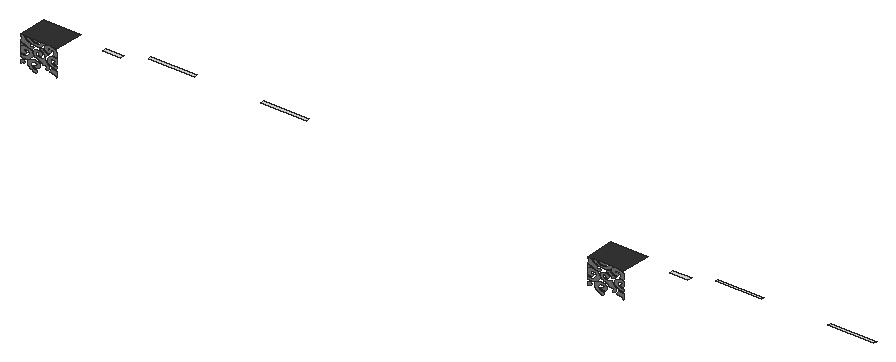
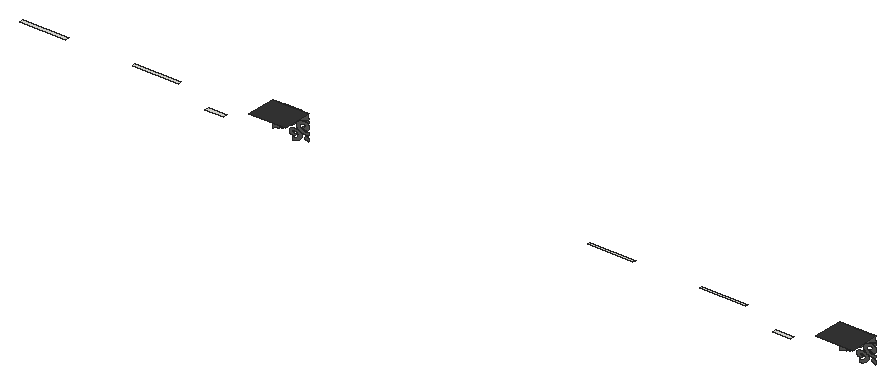
# SketchUp Ruby script. Lengths in inches.
U = 1.inch
M = Sketchup.active_model
def pt(a) = Geom::Point3d.new(a.map { |v| v * U })
def face(e, loops, mat)
  f = e.add_face(loops[0].map { |a| pt(a) })
  loops[1..].each { |l| e.add_face(l.map { |a| pt(a) }).erase! }
  f.material = f.back_material = mat if mat
  f
end
# faces: each face lists its corners as indices into pts; further lists are holes
def faces(e, pts, list, mat = nil) = list.each { |f| face(e, (f[0].is_a?(Array) ? f : [f]).map { |l| l.map { |i| pts[i] } }, mat) }
# xy, xz, yz: faces in a plane at the given z, y or x. An outline is a flat list of corners, or four numbers for a rectangle; further outlines are holes
def ring(l) = l.size == 4 ? [[l[0], l[1]], [l[2], l[1]], [l[2], l[3]], [l[0], l[3]]] : l.each_slice(2).to_a
def flat(e, list, mat, &to3) = list.each { |f| face(e, (f[0].is_a?(Array) ? f : [f]).map { |l| ring(l).map { |u, v| to3.(u, v) } }, mat) }
def xy(e, z, list, mat = nil) = flat(e, list, mat) { |x, y| [x, y, z] }
def xz(e, y, list, mat = nil) = flat(e, list, mat) { |x, z| [x, y, z] }
def yz(e, x, list, mat = nil) = flat(e, list, mat) { |y, z| [x, y, z] }
def lines(e, pts, list) = list.each { |a, b| e.add_line(pt(pts[a]), pt(pts[b])) }
# prism: a flat outline (further loops are holes) pulled along v
def prism(e, loops, v, mat = nil)
  f = face(e, loops, mat); d = Geom::Vector3d.new(v.map { |x| x * U })
  f.pushpull(f.normal.samedirection?(d) ? d.length : -d.length)
end
def box(e, o, s, mat = nil) = prism(e, [[o, [o[0] + s[0], o[1], o[2]], [o[0] + s[0], o[1] + s[1], o[2]], [o[0], o[1] + s[1], o[2]]]], [0, 0, s[2]], mat)
def at(x, y, z, deg = 0) = Geom::Transformation.translation(pt([x, y, z])) * Geom::Transformation.rotation(ORIGIN, Z_AXIS, deg.degrees)
def axes(o, x, y, z) = Geom::Transformation.new([*x, 0, *y, 0, *z, 0, *pt(o).to_a, 1])
def part(name) = M.definitions.add(name)
# library, detail: a bought-in or finely detailed component or shape, given as its bounding box
def library(name, o, s) = part(name).tap { |d| box(d.entities, o, s) }
def detail(e, o, s) = box(e.add_group.entities, o, s)
def put(e, d, t, mat = nil) = e.add_instance(d, t).tap { |i| i.material = mat if mat }
def group(e, t, mat = nil) = e.add_group.tap { |g| g.transformation = t; g.material = mat if mat }.entities
root = M.entities
M.materials.add("[0043_SaddleBrown]4").color = [124, 123, 122]
M.materials.add("[Slate Light Tile]").color = [54, 54, 54]
xy(root,742.22,[[496.1,656.57,535.93,665.86],[1746.73,656.57,1786.56,665.86]])
xy(root,759.44,[[367.98,589.17,449.07,653.8],[1618.6,589.17,1699.7,653.8]],"[Slate Light Tile]")
xy(root,766.875,[[602.01,651.03,703.26,657.03],[849.76,651.03,951.01,657.03],[1852.64,651.03,1953.89,657.03],[2100.38,651.03,2201.63,657.03]])
xz(root,589.17,[[402.71,695.68,403.12,696.06,403.48,696.46,403.8,696.87,404.06,697.3,404.27,697.74,404.42,698.18,404.53,698.63,404.57,699.09,404.56,699.55,404.49,700,404.375,700.45,404.2,700.89,402.85,700.8,401.49,700.82,400.14,700.95,398.84,701.2,397.61,701.55,396.47,702,395.4375,702.55,394.54,703.18,393.8,703.88,393.21,704.64,392.81,705.43,392.58,706.26,392.22,707.04,391.99,707.83,391.9,708.64,391.95,709.45,392.14,710.26,392.47,711.04,392.94,711.8,393.54,712.52,394.25,713.2,395.09,713.83,396.03,714.4,397.06,714.91,398.01,715.25,399.06,715.47,400.15,715.57,401.26,715.54,402.33,715.38,403.34,715.1,404.24,714.71,405.01,714.21,405.61,713.64,406.02,713.01,406.24,712.35,406.24,711.67,406.15,711.33,405.99,711.01,405.76,710.7,405.47,710.42,405.11,710.16,404.7,709.93,404.24,709.74,403.74,709.59,403.22,709.49,402.68,709.43,402.125,709.41,401.58,709.4375,401,709.45,400.4375,709.39,399.91,709.25,399.45,709.03,399.09,708.76,398.83,708.45,398.69,708.11,398.6875,707.75,398.8125,707.41,399.0625,707.09,399.42,706.82,399.875,706.6,401.12,706.22,402.46,705.99,403.84,705.91,405.23,705.99,406.5625,706.22,407.81,706.6,408.93,707.11,409.87,707.73,410.62,708.45,411.14,709.24,411.42,710.08,411.44,710.93,411.5,711.96,411.32,712.99,410.92,713.99,410.29,714.95,409.46,715.85,408.43,716.67,407.23,717.39,405.88,718.01,404.41,718.51,402.84,718.875,401.2,719.11,399.52,719.2,397.1875,719.12,394.9,718.81,392.72,718.29,390.7,717.5625,388.89,716.65,387.34,715.58,386.07,714.375,385.125,713.0625,384.52,711.67,384.29,710.24,384.41,708.81,384.9,707.4,385.46,706.04,386.21,704.71,387.17,703.44,388.31,702.22,389.62,701.07,391.1,699.99,392.74,699.01,394.52,698.125,396.42,697.34,398.43,696.67,400.53,696.11],[1653.33,695.68,1653.74,696.06,1654.11,696.46,1654.42,696.87,1654.68,697.3,1654.89,697.74,1655.05,698.18,1655.15,698.63,1655.2,699.09,1655.19,699.55,1655.12,700,1655,700.45,1654.82,700.89,1653.47,700.8,1652.11,700.82,1650.77,700.95,1649.47,701.2,1648.23,701.55,1647.09,702,1646.0625,702.55,1645.17,703.18,1644.42,703.88,1643.84,704.64,1643.43,705.43,1643.21,706.26,1642.84,707.04,1642.61,707.83,1642.52,708.64,1642.57,709.45,1642.77,710.26,1643.1,711.04,1643.56,711.8,1644.16,712.52,1644.88,713.2,1645.71,713.83,1646.65,714.4,1647.68,714.91,1648.64,715.25,1649.68,715.47,1650.78,715.57,1651.88,715.54,1652.96,715.38,1653.97,715.1,1654.87,714.71,1655.63,714.21,1656.24,713.64,1656.65,713.01,1656.86,712.35,1656.87,711.67,1656.78,711.33,1656.62,711.01,1656.39,710.7,1656.09,710.42,1655.73,710.16,1655.32,709.93,1654.86,709.74,1654.37,709.59,1653.85,709.49,1653.3,709.43,1652.75,709.41,1652.2,709.4375,1651.63,709.45,1651.0625,709.39,1650.54,709.25,1650.08,709.03,1649.71,708.76,1649.45,708.45,1649.32,708.11,1649.3125,707.75,1649.4375,707.41,1649.6875,707.09,1650.05,706.82,1650.5,706.6,1651.75,706.22,1653.08,705.99,1654.47,705.91,1655.85,705.99,1657.1875,706.22,1658.44,706.6,1659.55,707.11,1660.5,707.73,1661.24,708.45,1661.76,709.24,1662.04,710.08,1662.07,710.93,1662.12,711.96,1661.95,712.99,1661.54,713.99,1660.92,714.95,1660.08,715.85,1659.06,716.67,1657.86,717.39,1656.51,718.01,1655.03,718.51,1653.46,718.875,1651.82,719.11,1650.15,719.2,1647.8125,719.12,1645.53,718.81,1643.35,718.29,1641.33,717.5625,1639.52,716.65,1637.96,715.58,1636.69,714.375,1635.75,713.0625,1635.15,711.67,1634.91,710.24,1635.04,708.81,1635.53,707.4,1636.08,706.04,1636.84,704.71,1637.79,703.44,1638.93,702.22,1640.25,701.07,1641.73,699.99,1643.37,699.01,1645.14,698.125,1647.04,697.34,1649.05,696.67,1651.16,696.11],[449.07,702.875,449.07,713.56,448.03,713.58,447,713.62,445.96,713.6875,444.9375,713.78,443.92,713.9,442.9,714.04,441.9,714.21,440.91,714.4,439.93,714.62,438.97,714.85,438.02,715.12,437.09,715.4,436.99,714.74,436.83,714.08,436.62,713.43,436.35,712.78,436.03,712.15,435.66,711.52,435.23,710.91,434.76,710.3125,434.24,709.73,433.67,709.16,433.05,708.61,432.39,708.09,434.04,708.18,435.7,708.17,437.35,708.05,438.98,707.83,440.55,707.51,442.07,707.1,443.51,706.59,444.86,705.99,446.1,705.32,447.23,704.57,448.22,703.75],[1699.7,702.875,1699.7,713.56,1698.66,713.58,1697.62,713.62,1696.59,713.6875,1695.5625,713.78,1694.54,713.9,1693.53,714.04,1692.53,714.21,1691.53,714.4,1690.56,714.62,1689.59,714.85,1688.65,715.12,1687.72,715.4,1687.61,714.74,1687.45,714.08,1687.24,713.43,1686.97,712.78,1686.65,712.15,1686.28,711.52,1685.86,710.91,1685.38,710.3125,1684.86,709.73,1684.29,709.16,1683.68,708.61,1683.01,708.09,1684.67,708.18,1686.33,708.17,1687.98,708.05,1689.6,707.83,1691.18,707.51,1692.7,707.1,1694.14,706.59,1695.48,705.99,1696.73,705.32,1697.85,704.57,1698.84,703.75],[368.68,702.96,369.2,703.5,369.79,704.02,370.45,704.5,371.17,704.95,371.94,705.36,372.77,705.73,373.65,706.0625,374.5625,706.35,375.51,706.58,376.49,706.77,377.49,706.91,378.51,707,378.09,707.42,377.71,707.85,377.36,708.29,377.05,708.74,376.78,709.2,376.55,709.67,376.36,710.15,376.21,710.63,376.11,711.12,376.04,711.61,376.01,712.1,376.03,712.59,375.33,712.37,374.64,712.13,373.97,711.88,373.31,711.62,372.67,711.34,372.05,711.04,371.44,710.74,370.85,710.42,370.28,710.09,369.73,709.75,369.19,709.39,368.68,709.02],
  [1619.31,702.96,1619.83,703.5,1620.42,704.02,1621.07,704.5,1621.79,704.95,1622.57,705.36,1623.4,705.73,1624.27,706.0625,1625.1875,706.35,1626.14,706.58,1627.12,706.77,1628.12,706.91,1629.13,707,1628.71,707.42,1628.33,707.85,1627.99,708.29,1627.68,708.74,1627.41,709.2,1627.18,709.67,1626.99,710.15,1626.84,710.63,1626.73,711.12,1626.66,711.61,1626.64,712.1,1626.65,712.59,1625.95,712.37,1625.27,712.13,1624.6,711.88,1623.94,711.62,1623.3,711.34,1622.67,711.04,1622.07,710.74,1621.48,710.42,1620.9,710.09,1620.35,709.75,1619.82,709.39,1619.31,709.02],[426.76,710.37,427.32,710.4,427.86,710.47,428.38,710.59,428.87,710.76,429.32,710.97,429.71,711.21,430.04,711.49,430.31,711.79,430.5,712.11,430.61,712.44,430.65,712.79,430.86,713.36,431.01,713.9375,431.09,714.52,431.09,715.1,431.03,715.6875,430.9,716.27,430.7,716.84,430.43,717.4,430.1,717.95,429.7,718.49,429.24,719,428.72,719.49,427.79,720.35,426.92,721.23,426.11,722.14,425.375,723.07,424.71,724.02,424.11,724.99,423.59,725.97,423.14,726.97,422.76,727.97,422.46,728.99,422.23,730.01,422.08,731.04,421.11,730.28,419.99,729.6,418.74,729.01,417.37,728.53,415.91,728.17,414.39,727.92,412.83,727.8,411.25,727.8,409.6875,727.93,408.17,728.18,406.71,728.55,405.35,729.04,404.375,729.5,403.51,730.03,402.76,730.625,402.14,731.27,401.66,731.97,401.33,732.69,401.16,733.4375,401.14,734.19,401.28,734.94,401.58,735.67,402.03,736.37,402.62,737.03,403.16,737.29,403.76,737.48,404.41,737.625,405.08,737.71,405.76,737.73,406.4375,737.68,407.1,737.58,407.73,737.41,408.31,737.19,408.83,736.92,409.28,736.6,409.64,736.25,409.52,736,409.4375,735.74,409.38,735.48,409.36,735.22,409.38,734.96,409.43,734.7,409.51,734.44,409.62,734.1875,409.77,733.94,409.94,733.7,410.15,733.48,410.39,733.26,410.62,733.09,410.89,732.95,411.2,732.83,411.53,732.75,411.88,732.7,412.24,732.68,412.59,732.7,412.94,732.75,413.27,732.83,413.58,732.95,413.85,733.09,414.08,733.26,414.76,733.94,415.23,734.69,415.49,735.48,415.52,736.28,415.33,737.07,414.92,737.83,414.3125,738.54,413.51,739.18,412.55,739.72,411.45,740.15,410.24,740.46,408.97,740.63,407.55,740.79,406.11,740.82,404.67,740.71,403.28,740.47,401.97,740.1,400.76,739.62,399.6875,739.02,398.77,738.34,398.04,737.58,397.5,736.75,397.17,735.89,397.0625,735,396.95,733.98,397.01,732.96,397.25,731.95,397.65,730.96,398.22,730,398.95,729.08,399.83,728.21,400.85,727.4,402,726.66,403.27,726,404.64,725.42,406.1,724.9375,407.49,724.49,408.83,723.99,410.1,723.43,411.3,722.82,412.43,722.15,413.49,721.44,414.45,720.68,415.33,719.89,416.11,719.05,416.79,718.19,417.38,717.3,417.86,716.38,418.53,716.7,419.27,716.95,420.07,717.14,420.89,717.27,421.74,717.32,422.59,717.31,423.42,717.22,424.24,717.0625,425,716.84,425.72,716.55,426.36,716.21,426.92,715.82,427.13,715.51,427.28,715.18,427.36,714.84,427.38,714.5,427.34,714.16,427.24,713.83,427.08,713.5,426.86,713.1875,426.58,712.89,426.25,712.62,425.875,712.37,425.45,712.15,425.22,712.02,425.04,711.86,424.91,711.6875,424.84,711.5,424.83,711.31,424.875,711.12,424.98,710.9375,425.15,710.77,425.36,710.63,425.61,710.52,425.9,710.4375,426.2,710.39],[1677.38,710.37,1677.94,710.4,1678.49,710.47,1679.01,710.59,1679.5,710.76,1679.94,710.97,1680.33,711.21,1680.67,711.49,1680.93,711.79,1681.12,712.11,1681.24,712.44,1681.27,712.79,1681.49,713.36,1681.63,713.9375,1681.71,714.52,1681.72,715.1,1681.66,715.6875,1681.52,716.27,1681.32,716.84,1681.06,717.4,1680.72,717.95,1680.33,718.49,1679.87,719,1679.35,719.49,1678.41,720.35,1677.54,721.23,1676.74,722.14,1676,723.07,1675.33,724.02,1674.74,724.99,1674.21,725.97,1673.76,726.97,1673.38,727.97,1673.08,728.99,1672.86,730.01,1672.7,731.04,1671.74,730.28,1670.62,729.6,1669.36,729.01,1667.99,728.53,1666.54,728.17,1665.01,727.92,1663.45,727.8,1661.875,727.8,1660.3125,727.93,1658.79,728.18,1657.34,728.55,1655.97,729.04,1655,729.5,1654.13,730.03,1653.38,730.625,1652.76,731.27,1652.29,731.97,1651.96,732.69,1651.78,733.4375,1651.77,734.19,1651.91,734.94,1652.2,735.67,1652.65,736.37,1653.24,737.03,1653.79,737.29,1654.39,737.48,1655.03,737.625,1655.7,737.71,1656.38,737.73,1657.0625,737.68,1657.72,737.58,1658.35,737.41,1658.93,737.19,1659.45,736.92,1659.9,736.6,1660.27,736.25,1660.15,736,1660.0625,735.74,1660.01,735.48,1659.99,735.22,1660,734.96,1660.05,734.7,1660.13,734.44,1660.25,734.1875,1660.39,733.94,1660.57,733.7,1660.78,733.48,1661.01,733.26,1661.25,733.09,1661.52,732.95,1661.82,732.83,1662.16,732.75,1662.5,732.7,1662.86,732.68,1663.22,732.7,1663.57,732.75,1663.9,732.83,1664.2,732.95,1664.48,733.09,1664.71,733.26,1665.38,733.94,1665.85,734.69,1666.11,735.48,1666.15,736.28,1665.96,737.07,1665.55,737.83,1664.9375,738.54,1664.14,739.18,1663.17,739.72,1662.07,740.15,1660.87,740.46,1659.59,740.63,1658.17,740.79,1656.73,740.82,1655.3,740.71,1653.91,740.47,1652.59,740.1,1651.39,739.62,1650.3125,739.02,1649.4,738.34,1648.66,737.58,1648.125,736.75,1647.8,735.89,1647.6875,735,1647.58,733.98,1647.64,732.96,1647.87,731.95,1648.28,730.96,1648.84,730,1649.57,729.08,1650.45,728.21,1651.47,727.4,1652.62,726.66,1653.89,726,1655.27,725.42,1656.73,724.9375,1658.12,724.49,1659.45,723.99,1660.72,723.43,1661.93,722.82,1663.06,722.15,1664.11,721.44,1665.08,720.68,1665.95,719.89,1666.74,719.05,1667.42,718.19,1668,717.3,1668.48,716.38,1669.16,716.7,1669.9,716.95,1670.69,717.14,1671.52,717.27,1672.36,717.32,1673.21,717.31,1674.05,717.22,1674.86,717.0625,1675.63,716.84,1676.34,716.55,1676.99,716.21,1677.55,715.82,1677.75,715.51,1677.9,715.18,1677.99,714.84,1678.01,714.5,1677.97,714.16,1677.87,713.83,1677.7,713.5,1677.48,713.1875,1677.21,712.89,1676.875,712.62,1676.5,712.37,1676.08,712.15,1675.85,712.02,1675.66,711.86,1675.53,711.6875,1675.46,711.5,1675.45,711.31,1675.5,711.12,1675.61,710.9375,1675.77,710.77,1675.99,710.63,1676.24,710.52,1676.52,710.4375,1676.83,710.39],[375.3,715.57,377.56,715.62,379.79,715.84,381.97,716.22,384.05,716.76,386.02,717.44,387.84,718.27,389.48,719.23,390.93,720.29,392.16,721.46,393.82,723.2,394.98,725.09,395.59,727.07,395.64,729.09,395.12,731.08,394.05,732.99,392.45,734.75,390.39,736.33,387.92,737.66,385.11,738.7,382.05,739.44,378.83,739.84,377.68,739.71,376.54,739.5,375.45,739.24,374.4,738.91,373.4,738.52,372.47,738.07,371.62,737.57,370.84,737.02,370.15,736.43,369.5625,735.81,369.07,735.15,368.68,734.46,368.68,727.58,369.21,726.8,369.99,726.12,370.98,725.54,372.13,725.1,373.41,724.81,374.76,724.6875,376.12,724.74,377.4375,724.95,378.66,725.33,379.72,725.85,380.59,726.5,381.23,727.24,381.32,727.41,381.375,727.6,381.38,727.79,381.34,727.97,381.26,728.15,381.13,728.32,380.97,728.48,380.76,728.62,380.53,728.74,380.27,728.84,379.99,728.91,379.7,728.96,378.97,728.89,378.24,728.89,377.51,728.98,376.83,729.15,376.21,729.4,375.67,729.71,375.24,730.08,374.92,730.48,374.74,730.92,374.68,731.375,374.76,731.82,374.98,732.26,375.16,732.82,375.49,733.36,375.94,733.86,376.52,734.3,377.21,734.69,377.99,735.01,378.84,735.24,379.74,735.4,380.67,735.46,381.6,735.43,382.51,735.3125,383.39,735.11,384.74,734.44,385.93,733.66,386.93,732.78,387.71,731.83,388.27,730.81,388.59,729.76,388.66,728.7,388.49,727.63,388.07,726.59,387.42,725.6,386.54,724.68,385.47,723.84,385.03,723.28,384.51,722.75,383.93,722.25,383.28,721.77,382.57,721.34,381.81,720.9375,380.99,720.58,380.12,720.26,379.22,719.99,378.28,719.77,377.32,719.59,376.33,719.47,375.63,719.42,374.92,719.4,374.22,719.42,373.52,719.48,372.83,719.58,372.15,719.7,371.5,719.87,370.87,720.0625,370.27,720.29,369.7,720.55,369.17,720.84,368.68,721.15,368.68,716.4,370.83,715.96,373.04,715.68],[1625.92,715.57,1628.18,715.62,1630.42,715.84,1632.59,716.22,1634.68,716.76,1636.64,717.44,1638.46,718.27,1640.11,719.23,1641.55,720.29,1642.78,721.46,1644.45,723.2,1645.61,725.09,1646.22,727.07,1646.26,729.09,1645.74,731.08,1644.67,732.99,1643.08,734.75,1641.02,736.33,1638.55,737.66,1635.74,738.7,1632.68,739.44,1629.46,739.84,1628.3,739.71,1627.17,739.5,1626.07,739.24,1625.02,738.91,1624.03,738.52,1623.1,738.07,1622.24,737.57,1621.47,737.02,1620.78,736.43,1620.1875,735.81,1619.7,735.15,1619.31,734.46,1619.31,727.58,1619.84,726.8,1620.61,726.12,1621.6,725.54,1622.76,725.1,1624.04,724.81,1625.39,724.6875,1626.75,724.74,1628.0625,724.95,1629.28,725.33,1630.35,725.85,1631.22,726.5,1631.86,727.24,1631.95,727.41,1632,727.6,1632,727.79,1631.97,727.97,1631.88,728.15,1631.76,728.32,1631.59,728.48,1631.39,728.62,1631.16,728.74,1630.9,728.84,1630.62,728.91,1630.32,728.96,1629.6,728.89,1628.86,728.89,1628.14,728.98,1627.46,729.15,1626.84,729.4,1626.3,729.71,1625.87,730.08,1625.55,730.48,1625.36,730.92,1625.31,731.375,1625.39,731.82,1625.6,732.26,1625.79,732.82,1626.11,733.36,1626.57,733.86,1627.15,734.3,1627.84,734.69,1628.62,735.01,1629.47,735.24,1630.37,735.4,1631.29,735.46,1632.23,735.43,1633.14,735.3125,1634.01,735.11,1635.37,734.44,1636.56,733.66,1637.55,732.78,1638.34,731.83,1638.89,730.81,1639.21,729.76,1639.28,728.7,1639.11,727.63,1638.69,726.59,1638.04,725.6,1637.17,724.68,1636.09,723.84,1635.65,723.28,1635.14,722.75,1634.56,722.25,1633.91,721.77,1633.2,721.34,1632.43,720.9375,1631.61,720.58,1630.75,720.26,1629.84,719.99,1628.91,719.77,1627.94,719.59,1626.96,719.47,1626.25,719.42,1625.55,719.4,1624.84,719.42,1624.14,719.48,1623.45,719.58,1622.78,719.7,1622.125,719.87,1621.49,720.0625,1620.89,720.29,1620.33,720.55,1619.8,720.84,1619.31,721.15,1619.31,716.4,1621.45,715.96,1623.67,715.68],
  [446.48,718.47,449.07,718.69,449.07,722.69,446.84,722.65,444.63,722.84,442.51,723.27,440.54,723.91,438.79,724.76,437.3,725.78,436.12,726.94,435.29,728.21,434.83,729.55,434.76,730.92,435.07,732.28,435.77,733.58,436.5625,734.14,437.52,734.59,438.59,734.93,439.75,735.14,440.95,735.21,442.15,735.13,443.31,734.93,444.38,734.59,445.33,734.13,446.125,733.57,446.73,732.93,447.13,732.23,447.21,731.95,447.2,731.66,447.11,731.375,446.95,731.11,446.71,730.86,446.41,730.64,446.05,730.46,445.65,730.3125,445.21,730.21,444.75,730.16,444.28,730.16,443.82,730.2,443.57,730.14,443.35,730.06,443.13,729.96,442.9375,729.85,442.76,729.73,442.61,729.6,442.48,729.45,442.38,729.3,442.3,729.15,442.26,728.99,442.24,728.83,442.24,728.67,442.61,728.34,443.05,728.04,443.55,727.78,444.1,727.5625,444.6875,727.39,445.31,727.27,445.95,727.2,446.6,727.1875,447.25,727.22,447.89,727.3125,448.5,727.45,449.07,727.64,449.07,737.55,448.01,738.08,446.86,738.51,445.62,738.86,444.32,739.11,442.99,739.26,441.63,739.32,440.28,739.26,438.94,739.11,437.65,738.86,436.41,738.51,435.25,738.08,434.19,737.55,433.3,737.02,432.47,736.46,431.69,735.86,430.99,735.23,430.36,734.57,429.8,733.89,429.32,733.18,428.91,732.46,428.58,731.72,428.34,730.97,428.18,730.22,428.1,729.45,428.21,727.85,428.72,726.27,429.61,724.75,430.86,723.34,432.44,722.06,434.32,720.94,436.45,720,438.79,719.27,441.27,718.77,443.86,718.5],[1697.1,718.47,1699.7,718.69,1699.7,722.69,1697.47,722.65,1695.26,722.84,1693.14,723.27,1691.17,723.91,1689.41,724.76,1687.92,725.78,1686.75,726.94,1685.91,728.21,1685.45,729.55,1685.38,730.92,1685.7,732.28,1686.39,733.58,1687.1875,734.14,1688.14,734.59,1689.22,734.93,1690.375,735.14,1691.58,735.21,1692.78,735.13,1693.94,734.93,1695.01,734.59,1695.96,734.13,1696.75,733.57,1697.36,732.93,1697.76,732.23,1697.83,731.95,1697.82,731.66,1697.74,731.375,1697.57,731.11,1697.34,730.86,1697.03,730.64,1696.68,730.46,1696.27,730.3125,1695.83,730.21,1695.37,730.16,1694.9,730.16,1694.44,730.2,1694.2,730.14,1693.97,730.06,1693.76,729.96,1693.5625,729.85,1693.39,729.73,1693.24,729.6,1693.11,729.45,1693.01,729.3,1692.93,729.15,1692.88,728.99,1692.86,728.83,1692.87,728.67,1693.24,728.34,1693.67,728.04,1694.17,727.78,1694.72,727.5625,1695.3125,727.39,1695.93,727.27,1696.57,727.2,1697.23,727.1875,1697.875,727.22,1698.51,727.3125,1699.12,727.45,1699.7,727.64,1699.7,737.55,1698.64,738.08,1697.48,738.51,1696.24,738.86,1694.95,739.11,1693.61,739.26,1692.26,739.32,1690.9,739.26,1689.57,739.11,1688.27,738.86,1687.04,738.51,1685.88,738.08,1684.82,737.55,1683.92,737.02,1683.09,736.46,1682.32,735.86,1681.62,735.23,1680.98,734.57,1680.42,733.89,1679.94,733.18,1679.54,732.46,1679.21,731.72,1678.96,730.97,1678.8,730.22,1678.72,729.45,1678.84,727.85,1679.35,726.27,1680.24,724.75,1681.49,723.34,1683.07,722.06,1684.94,720.94,1687.08,720,1689.41,719.27,1691.9,718.77,1694.48,718.5],[423.18,735.95,423.73,736.35,424.29,736.73,424.86,737.11,425.44,737.49,426.04,737.86,426.64,738.22,427.25,738.57,427.87,738.93,429.13,739.61,429.78,739.94,430.4375,740.26,428.78,740.53,427.17,740.9,425.625,741.37,424.16,741.92,422.8,742.5625,421.54,743.28,420.4,744.07,419.4,744.93,418.54,745.84,417.83,746.8,417.27,747.8,416.88,748.83,416.4,748.48,415.89,748.14,415.37,747.82,414.83,747.5,414.27,747.2,413.69,746.92,413.09,746.64,412.48,746.38,411.86,746.13,411.22,745.9,410.56,745.68,409.89,745.48,411.46,744.99,412.96,744.43,414.39,743.8125,415.75,743.13,417.03,742.39,418.22,741.6,419.3125,740.76,420.3,739.87,421.19,738.94,421.97,737.98,422.63,736.98],[1673.8,735.95,1674.35,736.35,1675.49,737.11,1676.07,737.49,1676.66,737.86,1677.26,738.22,1677.87,738.57,1678.49,738.93,1679.12,739.27,1679.76,739.61,1680.41,739.94,1681.0625,740.26,1679.4,740.53,1677.79,740.9,1676.25,741.37,1674.79,741.92,1673.42,742.5625,1672.16,743.28,1671.03,744.07,1670.03,744.93,1669.16,745.84,1668.45,746.8,1667.9,747.8,1667.5,748.83,1667.02,748.48,1666.52,748.14,1666,747.82,1665.45,747.5,1664.89,747.2,1664.31,746.92,1663.72,746.64,1663.11,746.38,1662.48,746.13,1661.84,745.9,1661.19,745.68,1660.52,745.48,1662.08,744.99,1663.58,744.43,1665.02,743.8125,1666.38,743.13,1667.66,742.39,1668.84,741.6,1669.9375,740.76,1670.93,739.87,1671.82,738.94,1672.59,737.98,1673.26,736.98],[368.68,739.1,369.1,739.38,369.54,739.65,369.99,739.92,370.46,740.16,370.96,740.4,371.46,740.62,371.99,740.83,372.52,741.02,373.08,741.2,373.64,741.36,374.21,741.51,374.8,741.64,374.42,741.93,374.01,742.19,373.57,742.4375,373.1,742.66,372.61,742.87,372.09,743.06,371.56,743.22,371.01,743.36,370.4375,743.47,369.86,743.5625,369.28,743.63,368.68,743.67],
  [1619.31,739.1,1619.72,739.38,1620.16,739.65,1620.62,739.92,1621.09,740.16,1621.58,740.4,1622.09,740.62,1622.61,740.83,1623.15,741.02,1623.7,741.2,1624.26,741.36,1624.84,741.51,1625.42,741.64,1625.04,741.93,1624.63,742.19,1624.19,742.4375,1623.72,742.66,1623.23,742.87,1622.72,743.06,1622.18,743.22,1621.63,743.36,1621.0625,743.47,1620.49,743.5625,1619.9,743.63,1619.31,743.67],[390.73,739.72,391.66,739.75,392.56,739.85,393.45,740,394.31,740.21,394.61,740.31,394.9,740.42,395.18,740.55,395.43,740.6875,395.67,740.84,395.88,741,396.08,741.18,396.24,741.36,396.39,741.55,396.5,741.75,396.59,741.95,396.65,742.16,396.67,742.37,396.66,742.57,396.61,742.77,396.52,742.97,396.4,743.16,396.24,743.34,396.05,743.51,395.83,743.66,395.58,743.8,395.3125,743.92,395.02,744.02,394.71,744.09,394.52,743.88,394.1,743.48,393.87,743.28,393.63,743.09,393.38,742.9,393.125,742.72,392.85,742.54,392.58,742.375,392.29,742.21,391.99,742.05,391.68,741.9,391.26,741.96,390.84,742.04,390.44,742.15,390.06,742.28,389.71,742.43,389.375,742.6,389.07,742.79,388.8,743,388.5625,743.23,388.36,743.46,388.2,743.71,388.08,743.97,387.94,744.37,387.83,744.78,387.75,745.18,387.7,745.6,387.69,746.01,387.71,746.42,387.77,746.83,387.86,747.24,387.97,747.64,388.125,748.04,388.31,748.4375,388.52,748.83,387.06,749.17,385.64,749.6,384.3,750.09,383.03,750.66,381.85,751.3,380.76,752,379.78,752.76,378.92,753.5625,378.18,754.41,377.56,755.3,377.07,756.22,376.72,757.16,376.34,757.31,375.96,757.47,375.6,757.63,375.24,757.81,374.89,757.99,374.56,758.17,374.23,758.36,373.91,758.5625,373.6,758.77,373.3,758.98,373.01,759.19,372.73,759.44,368.68,759.44,368.68,758.69,369.77,757.9375,370.6875,757.1,371.42,756.2,371.95,755.24,372.27,754.26,372.375,753.25,372.27,752.24,371.95,751.25,371.42,750.3,370.6875,749.4,369.77,748.56,368.68,747.8,368.68,746.79,370.16,746.6,371.61,746.36,373.04,746.08,374.44,745.74,375.8125,745.36,377.15,744.93,378.44,744.46,379.69,743.95,380.89,743.39,382.04,742.79,383.14,742.16,384.18,741.49,384.83,741.09,385.55,740.73,386.32,740.43,387.14,740.17,388.01,739.97,388.9,739.83,389.8125,739.74],[1641.36,739.72,1642.28,739.75,1643.19,739.85,1644.08,740,1644.93,740.21,1645.24,740.31,1645.53,740.42,1645.8,740.55,1646.06,740.6875,1646.29,740.84,1646.51,741,1646.7,741.18,1646.87,741.36,1647.01,741.55,1647.125,741.75,1647.21,741.95,1647.27,742.16,1647.3,742.37,1647.29,742.57,1647.24,742.77,1647.15,742.97,1647.03,743.16,1646.87,743.34,1646.68,743.51,1646.46,743.66,1646.21,743.8,1645.9375,743.92,1645.65,744.02,1645.34,744.09,1645.14,743.88,1644.94,743.68,1644.5,743.28,1644.26,743.09,1644.01,742.9,1643.75,742.72,1643.48,742.54,1643.2,742.375,1642.91,742.21,1642.61,742.05,1642.31,741.9,1641.88,741.96,1641.47,742.04,1641.07,742.15,1640.69,742.28,1640.33,742.43,1640,742.6,1639.7,742.79,1639.43,743,1639.1875,743.23,1638.99,743.46,1638.82,743.71,1638.7,743.97,1638.56,744.37,1638.45,744.78,1638.375,745.18,1638.33,745.6,1638.32,746.01,1638.34,746.42,1638.39,746.83,1638.48,747.24,1638.6,747.64,1638.75,748.04,1638.93,748.4375,1639.15,748.83,1637.68,749.17,1636.27,749.6,1634.92,750.09,1633.65,750.66,1632.47,751.3,1631.39,752,1630.41,752.76,1629.54,753.5625,1628.8,754.41,1628.18,755.3,1627.69,756.22,1627.34,757.16,1626.96,757.31,1626.22,757.63,1625.52,757.99,1625.18,758.17,1624.85,758.36,1624.53,758.5625,1624.22,758.77,1623.92,758.98,1623.63,759.19,1623.35,759.44,1619.31,759.44,1619.31,758.69,1620.39,757.9375,1621.3125,757.1,1622.04,756.2,1622.57,755.24,1622.89,754.26,1623,753.25,1622.89,752.24,1622.57,751.25,1622.04,750.3,1621.3125,749.4,1620.39,748.56,1619.31,747.8,1619.31,746.79,1620.78,746.6,1622.23,746.36,1623.67,746.08,1625.07,745.74,1626.4375,745.36,1627.77,744.93,1629.07,744.46,1630.32,743.95,1631.52,743.39,1632.67,742.79,1633.76,742.16,1634.8,741.49,1635.45,741.09,1636.17,740.73,1636.95,740.43,1637.77,740.17,1638.63,739.97,1639.53,739.83,1640.4375,739.74],[449.07,741.3,449.07,748.98,448.66,750.12,448.07,751.22,447.3,752.29,446.38,753.3,445.3,754.26,444.07,755.15,442.71,755.96,441.23,756.6875,439.64,757.32,437.96,757.86,436.21,758.3,434.39,758.63,432.72,758.68,431.0625,758.58,429.44,758.33,427.9,757.93,426.48,757.4,425.2,756.74,424.09,755.98,423.18,755.12,422.48,754.18,422.02,753.2,421.8,752.18,421.83,751.16,421.79,750.51,421.87,749.86,422.08,749.23,422.41,748.61,422.86,748.03,423.43,747.48,424.09,746.98,424.86,746.53,425.7,746.14,426.62,745.82,427.59,745.57,428.61,745.39,429.29,745.15,430.02,744.97,430.79,744.88,431.58,744.87,432.36,744.94,433.11,745.09,433.8,745.32,434.42,745.62,434.95,745.97,435.375,746.38,435.68,746.83,435.86,747.3,436.25,747.65,436.55,748.03,436.73,748.4375,436.8,748.86,436.75,749.29,436.58,749.7,436.29,750.08,435.9,750.4375,435.42,750.74,434.86,750.99,434.24,751.18,433.58,751.3,433.1,750.88,432.85,750.68,432.58,750.49,432.3,750.3,432.02,750.12,431.72,749.9375,431.42,749.77,431.1,749.6,430.78,749.44,430.45,749.29,430.11,749.15,429.74,749.29,429.39,749.46,429.08,749.65,428.8,749.86,428.5625,750.09,428.36,750.33,428.21,750.58,428.1,750.84,428.04,751.11,428.02,751.38,428.06,751.65,428.14,751.92,428.42,752.45,428.85,752.95,429.4,753.4,430.06,753.79,430.81,754.11,431.64,754.36,432.52,754.51,433.43,754.58,434.34,754.56,435.24,754.44,436.09,754.24,436.89,753.96,438.3,753.26,439.55,752.46,440.61,751.55,441.47,750.57,442.1,749.53,442.49,748.44,442.64,747.33,442.55,746.22,442.21,745.125,441.63,744.07,440.83,743.07,439.81,742.15,440.6,742.26,441.39,742.34,442.1875,742.39,442.99,742.4,443.79,742.38,444.59,742.32,445.38,742.24,446.16,742.11,446.92,741.96,447.66,741.77,448.38,741.55],[1699.7,741.3,1699.7,748.98,1699.28,750.12,1698.69,751.22,1697.93,752.29,1697,753.3,1695.92,754.26,1694.7,755.15,1693.34,755.96,1691.86,756.6875,1690.27,757.32,1688.59,757.86,1686.83,758.3,1685.01,758.63,1683.35,758.68,1681.6875,758.58,1680.07,758.33,1678.53,757.93,1677.1,757.4,1675.82,756.74,1674.71,755.98,1673.8,755.12,1673.11,754.18,1672.65,753.2,1672.43,752.18,1672.46,751.16,1672.41,750.51,1672.49,749.86,1672.7,749.23,1673.03,748.61,1673.49,748.03,1674.05,747.48,1674.72,746.98,1675.48,746.53,1676.33,746.14,1677.25,745.82,1678.22,745.57,1679.24,745.39,1679.91,745.15,1680.65,744.97,1681.42,744.88,1682.21,744.87,1682.98,744.94,1683.73,745.09,1684.42,745.32,1685.05,745.62,1685.58,745.97,1686,746.38,1686.3,746.83,1686.48,747.3,1686.88,747.65,1687.18,748.03,1687.36,748.4375,1687.43,748.86,1687.37,749.29,1687.2,749.7,1686.92,750.08,1686.53,750.4375,1686.05,750.74,1685.49,750.99,1684.87,751.18,1684.2,751.3,1683.97,751.09,1683.73,750.88,1683.47,750.68,1683.21,750.49,1682.93,750.3,1682.64,750.12,1682.35,749.9375,1682.04,749.77,1681.73,749.6,1681.41,749.44,1681.07,749.29,1680.74,749.15,1680.36,749.29,1680.02,749.46,1679.7,749.65,1679.43,749.86,1679.1875,750.09,1678.99,750.33,1678.83,750.58,1678.73,750.84,1678.66,751.11,1678.65,751.38,1678.68,751.65,1678.76,751.92,1679.05,752.45,1679.47,752.95,1680.02,753.4,1680.68,753.79,1681.43,754.11,1682.26,754.36,1683.14,754.51,1684.05,754.58,1684.97,754.56,1685.86,754.44,1686.72,754.24,1687.51,753.96,1688.93,753.26,1690.18,752.46,1691.24,751.55,1692.09,750.57,1692.72,749.53,1693.12,748.44,1693.27,747.33,1693.17,746.22,1692.83,745.125,1692.26,744.07,1691.45,743.07,1690.44,742.15,1691.22,742.26,1692.01,742.34,1692.8125,742.39,1693.61,742.4,1694.42,742.38,1695.21,742.32,1696,742.24,1696.78,742.11,1697.54,741.96,1698.28,741.77,1699,741.55],
  [401.92,748.82,406.74,749.18,411.3,750.2,415.35,751.84,418.6875,754.01,421.12,756.6,422.52,759.44,416.36,759.44,415.18,757.58,413.375,755.92,411.02,754.53,408.24,753.48,405.15,752.83,401.91,752.61,398.67,752.81,395.57,753.45,392.77,754.48,390.4,755.85,388.57,757.51,387.36,759.44,381.2,759.44,382.63,756.52,385.09,753.95,388.45,751.79,392.52,750.17,397.09,749.16],[1652.54,748.82,1657.36,749.18,1661.92,750.2,1665.98,751.84,1669.3125,754.01,1671.74,756.6,1673.15,759.44,1666.99,759.44,1665.81,757.58,1664,755.92,1661.65,754.53,1658.86,753.48,1655.78,752.83,1652.54,752.61,1649.29,752.81,1646.2,753.45,1643.4,754.48,1641.02,755.85,1639.19,757.51,1637.98,759.44,1631.83,759.44,1633.26,756.52,1635.72,753.95,1639.07,751.79,1643.14,750.17,1647.71,749.16],[402.23,756.12,403.99,756.22,405.69,756.52,407.27,757.02,408.67,757.6875,409.83,758.51,410.73,759.44,393.73,759.44,394.63,758.51,395.8,757.6875,397.19,757.02,398.77,756.52,400.47,756.22],[1652.86,756.12,1654.62,756.22,1656.32,756.52,1657.9,757.02,1659.29,757.6875,1660.46,758.51,1661.35,759.44,1644.36,759.44,1645.25,758.51,1646.42,757.6875,1647.82,757.02,1649.39,756.52,1651.09,756.22]],"[0043_SaddleBrown]4")
p = [[431.98,589.17,696.8],[431.89,589.17,696.34],[368.68,589.17,746.79],[368.68,589.17,743.67],[1682.6,589.17,696.8],[1682.52,589.17,696.34],
  [1619.31,589.17,746.79],[1619.31,589.17,743.67]]
lines(root,p,[[0,1],[2,3],[4,5],[6,7]])
